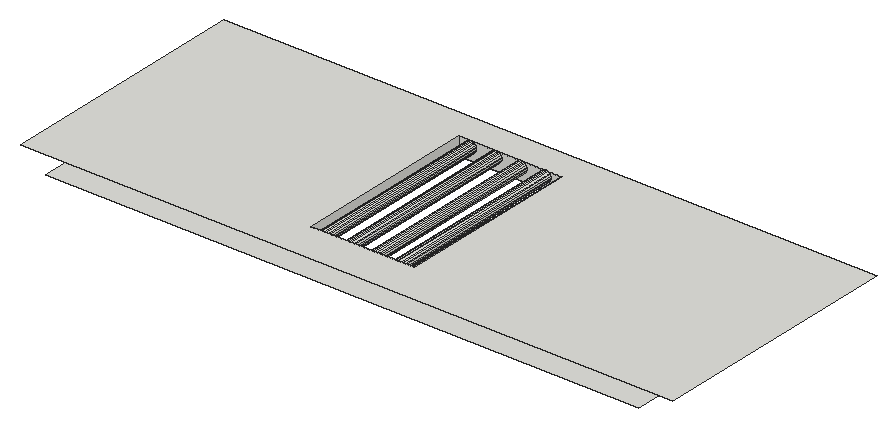
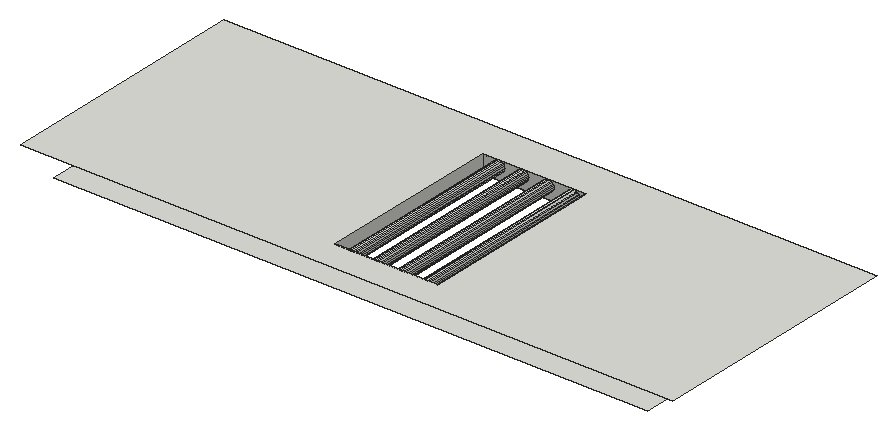
# SketchUp Ruby script. Lengths in inches.
U = 1.inch
M = Sketchup.active_model
def pt(a) = Geom::Point3d.new(a.map { |v| v * U })
def face(e, loops, mat)
  f = e.add_face(loops[0].map { |a| pt(a) })
  loops[1..].each { |l| e.add_face(l.map { |a| pt(a) }).erase! }
  f.material = f.back_material = mat if mat
  f
end
# faces: each face lists its corners as indices into pts; further lists are holes
def faces(e, pts, list, mat = nil) = list.each { |f| face(e, (f[0].is_a?(Array) ? f : [f]).map { |l| l.map { |i| pts[i] } }, mat) }
# xy, xz, yz: faces in a plane at the given z, y or x. An outline is a flat list of corners, or four numbers for a rectangle; further outlines are holes
def ring(l) = l.size == 4 ? [[l[0], l[1]], [l[2], l[1]], [l[2], l[3]], [l[0], l[3]]] : l.each_slice(2).to_a
def flat(e, list, mat, &to3) = list.each { |f| face(e, (f[0].is_a?(Array) ? f : [f]).map { |l| ring(l).map { |u, v| to3.(u, v) } }, mat) }
def xy(e, z, list, mat = nil) = flat(e, list, mat) { |x, y| [x, y, z] }
def xz(e, y, list, mat = nil) = flat(e, list, mat) { |x, z| [x, y, z] }
def yz(e, x, list, mat = nil) = flat(e, list, mat) { |y, z| [x, y, z] }
def lines(e, pts, list) = list.each { |a, b| e.add_line(pt(pts[a]), pt(pts[b])) }
# prism: a flat outline (further loops are holes) pulled along v
def prism(e, loops, v, mat = nil)
  f = face(e, loops, mat); d = Geom::Vector3d.new(v.map { |x| x * U })
  f.pushpull(f.normal.samedirection?(d) ? d.length : -d.length)
end
def box(e, o, s, mat = nil) = prism(e, [[o, [o[0] + s[0], o[1], o[2]], [o[0] + s[0], o[1] + s[1], o[2]], [o[0], o[1] + s[1], o[2]]]], [0, 0, s[2]], mat)
def at(x, y, z, deg = 0) = Geom::Transformation.translation(pt([x, y, z])) * Geom::Transformation.rotation(ORIGIN, Z_AXIS, deg.degrees)
def axes(o, x, y, z) = Geom::Transformation.new([*x, 0, *y, 0, *z, 0, *pt(o).to_a, 1])
def part(name) = M.definitions.add(name)
# library, detail: a bought-in or finely detailed component or shape, given as its bounding box
def library(name, o, s) = part(name).tap { |d| box(d.entities, o, s) }
def detail(e, o, s) = box(e.add_group.entities, o, s)
def put(e, d, t, mat = nil) = e.add_instance(d, t).tap { |i| i.material = mat if mat }
def group(e, t, mat = nil) = e.add_group.tap { |g| g.transformation = t; g.material = mat if mat }.entities
root = M.entities
xy(root,367.15,[[[9.02,53.875,221.54,144.86],[92.68,68.23,129.5,134.29],[86.02,110.58,86.54,110.6,87.04,110.74,87.48,111.01,87.84,111.39,88.09,111.85,88.22,112.36,88.2,112.88,88.06,113.38,87.79,113.83,87.41,114.1875,86.95,114.4375,86.44,114.56,85.92,114.55,85.42,114.4,84.97,114.13,84.61,113.75,84.36,113.29,84.24,112.78,84.25,112.26,84.4,111.76,84.67,111.32,85.05,110.96,85.51,110.71],[86.02,126.33,86.54,126.35,87.04,126.49,87.48,126.76,87.84,127.14,88.09,127.6,88.22,128.11,88.2,128.63,88.06,129.13,87.79,129.58,87.41,129.9375,86.95,130.1875,86.44,130.31,85.92,130.3,85.42,130.15,84.97,129.88,84.61,129.5,84.36,129.04,84.24,128.53,84.25,128.01,84.4,127.51,84.67,127.07,85.05,126.71,85.51,126.46],[86.02,95.96,86.54,95.97,87.04,96.12,87.48,96.39,87.84,96.77,88.09,97.23,88.22,97.73,88.2,98.26,88.06,98.76,87.79,99.2,87.41,99.5625,86.95,99.8125,86.44,99.94,85.92,99.92,85.42,99.78,84.97,99.5,84.61,99.125,84.36,98.67,84.24,98.16,84.25,97.64,84.4,97.14,84.67,96.69,85.05,96.33,85.51,96.08],[86.02,85.02,86.54,85.03,87.04,85.18,87.48,85.45,87.84,85.83,88.09,86.29,88.22,86.8,88.2,87.32,88.06,87.82,87.79,88.26,87.41,88.625,86.95,88.875,86.44,89,85.92,88.99,85.42,88.84,84.97,88.57,84.61,88.1875,84.36,87.73,84.24,87.22,84.25,86.7,84.4,86.2,84.67,85.75,85.05,85.39,85.51,85.14],[86.02,73.4,86.54,73.41,87.04,73.56,87.48,73.83,87.84,74.21,88.09,74.66,88.22,75.17,88.2,75.69,88.06,76.19,87.79,76.64,87.41,77,86.95,77.25,86.44,77.37,85.92,77.36,85.42,77.21,84.97,76.94,84.61,76.5625,84.36,76.1,84.24,75.6,84.25,75.08,84.4,74.57,84.67,74.13,85.05,73.77,85.51,73.52],[144.73,72.4,145.25,72.41,145.75,72.56,146.2,72.83,146.56,73.21,146.81,73.67,146.93,74.17,146.92,74.7,146.77,75.2,146.5,75.64,146.12,76,145.66,76.25,145.16,76.375,144.63,76.36,144.13,76.22,143.6875,75.94,143.33,75.57,143.08,75.11,142.95,74.6,142.97,74.08,143.11,73.58,143.39,73.13,143.76,72.77,144.22,72.52],[144.73,90.84,145.25,90.85,145.75,91,146.2,91.27,146.56,91.65,146.81,92.1,146.93,92.61,146.92,93.13,146.77,93.64,146.5,94.08,146.12,94.44,145.66,94.69,145.16,94.8125,144.63,94.8,144.13,94.65,143.6875,94.38,143.33,94,143.08,93.55,142.95,93.04,142.97,92.52,143.11,92.01,143.39,91.57,143.76,91.21,144.22,90.96],[144.73,112.15,145.25,112.16,145.75,112.31,146.2,112.58,146.56,112.96,146.81,113.42,146.93,113.92,146.92,114.45,146.77,114.95,146.5,115.39,146.12,115.75,145.66,116,145.16,116.125,144.63,116.11,144.13,115.97,143.6875,115.69,143.33,115.32,143.08,114.86,142.95,114.35,142.97,113.83,143.11,113.33,143.39,112.88,143.76,112.52,144.22,112.27],[144.73,130.65,145.25,130.66,145.75,130.81,146.2,131.08,146.56,131.46,146.81,131.92,146.93,132.42,146.92,132.95,146.77,133.45,146.5,133.89,146.12,134.25,145.66,134.5,145.16,134.625,144.63,134.61,144.13,134.47,143.6875,134.19,143.33,133.82,143.08,133.36,142.95,132.85,142.97,132.33,143.11,131.83,143.39,131.38,143.76,131.02,144.22,130.77]],[86.02,126.33,85.51,126.46,85.05,126.71,84.67,127.07,84.4,127.51,84.25,128.01,84.24,128.53,84.36,129.04,84.61,129.5,84.97,129.88,85.42,130.15,85.92,130.3,86.44,130.31,86.95,130.1875,87.41,129.9375,87.79,129.58,88.06,129.13,88.2,128.63,88.22,128.11,88.09,127.6,87.84,127.14,87.48,126.76,87.04,126.49,86.54,126.35]])
xy(root,367.77,[[144.73,112.15,144.22,112.27,143.76,112.52,143.39,112.88,143.11,113.33,142.97,113.83,142.95,114.35,143.08,114.86,143.33,115.32,143.6875,115.69,144.13,115.97,144.63,116.11,145.16,116.125,145.66,116,146.12,115.75,146.5,115.39,146.77,114.95,146.92,114.45,146.93,113.92,146.81,113.42,146.56,112.96,146.2,112.58,145.75,112.31,145.25,112.16],[144.73,130.65,144.22,130.77,143.76,131.02,143.39,131.38,143.11,131.83,142.97,132.33,142.95,132.85,143.08,133.36,143.33,133.82,143.6875,134.19,144.13,134.47,144.63,134.61,145.16,134.625,145.66,134.5,146.12,134.25,146.5,133.89,146.77,133.45,146.92,132.95,146.93,132.42,146.81,131.92,146.56,131.46,146.2,131.08,145.75,130.81,145.25,130.66]])
xy(root,368.02,[[86.02,85.02,85.51,85.14,85.05,85.39,84.67,85.75,84.4,86.2,84.25,86.7,84.24,87.22,84.36,87.73,84.61,88.1875,84.97,88.57,85.42,88.84,85.92,88.99,86.44,89,86.95,88.875,87.41,88.625,87.79,88.26,88.06,87.82,88.2,87.32,88.22,86.8,88.09,86.29,87.84,85.83,87.48,85.45,87.04,85.18,86.54,85.03]])
xy(root,368.27,[[86.02,95.96,85.51,96.08,85.05,96.33,84.67,96.69,84.4,97.14,84.25,97.64,84.24,98.16,84.36,98.67,84.61,99.125,84.97,99.5,85.42,99.78,85.92,99.92,86.44,99.94,86.95,99.8125,87.41,99.5625,87.79,99.2,88.06,98.76,88.2,98.26,88.22,97.73,88.09,97.23,87.84,96.77,87.48,96.39,87.04,96.12,86.54,95.97]])
xy(root,368.34,[[86.02,73.4,85.51,73.52,85.05,73.77,84.67,74.13,84.4,74.57,84.25,75.08,84.24,75.6,84.36,76.1,84.61,76.5625,84.97,76.94,85.42,77.21,85.92,77.36,86.44,77.37,86.95,77.25,87.41,77,87.79,76.64,88.06,76.19,88.2,75.69,88.22,75.17,88.09,74.66,87.84,74.21,87.48,73.83,87.04,73.56,86.54,73.41]])
xy(root,368.65,[[144.73,90.84,144.22,90.96,143.76,91.21,143.39,91.57,143.11,92.01,142.97,92.52,142.95,93.04,143.08,93.55,143.33,94,143.6875,94.38,144.13,94.65,144.63,94.8,145.16,94.8125,145.66,94.69,146.12,94.44,146.5,94.08,146.77,93.64,146.92,93.13,146.93,92.61,146.81,92.1,146.56,91.65,146.2,91.27,145.75,91,145.25,90.85]])
xy(root,369.46,[[86.02,110.58,85.51,110.71,85.05,110.96,84.67,111.32,84.4,111.76,84.25,112.26,84.24,112.78,84.36,113.29,84.61,113.75,84.97,114.13,85.42,114.4,85.92,114.55,86.44,114.56,86.95,114.4375,87.41,114.1875,87.79,113.83,88.06,113.38,88.2,112.88,88.22,112.36,88.09,111.85,87.84,111.39,87.48,111.01,87.04,110.74,86.54,110.6]])
xy(root,373.61,[[[0,53.875,233.71,144.86],[92.68,68.23,129.5,134.29]]])
xz(root,68.23,[[[92.68,367.15,129.5,373.61],[123.71,369.61,124.23,369.68,124.71,369.88,125.12,370.21,125.43,370.62,125.63,371.11,125.69,371.625,125.62,372.14,125.41,372.62,125.09,373.03,124.68,373.35,124.19,373.54,123.67,373.61,123.16,373.53,122.68,373.33,122.26,373.01,121.95,372.59,121.76,372.11,121.69,371.59,121.76,371.07,121.97,370.59,122.29,370.18,122.71,369.87,123.19,369.67]]])
xz(root,134.29,[[[92.68,367.15,129.5,373.61],[123.71,369.61,123.19,369.67,122.71,369.87,122.29,370.18,121.97,370.59,121.76,371.07,121.69,371.59,121.76,372.11,121.95,372.59,122.26,373.01,122.68,373.33,123.16,373.53,123.67,373.61,124.19,373.54,124.68,373.35,125.09,373.03,125.41,372.62,125.62,372.14,125.69,371.625,125.63,371.11,125.43,370.62,125.12,370.21,124.71,369.88,124.23,369.68]]])
yz(root,92.68,[[68.23,367.15,134.29,373.61]])
yz(root,129.5,[[68.23,367.15,134.29,373.61]])
p = [[86.02,73.4,367.15],[85.51,73.52,367.15],[85.51,73.52,368.34],[86.02,73.4,368.34],[86.54,73.41,367.15],[86.54,73.41,368.34],
  [87.04,73.56,367.15],[87.04,73.56,368.34],[85.05,73.77,367.15],[85.05,73.77,368.34],[87.48,73.83,367.15],[87.48,73.83,368.34],
  [84.67,74.13,367.15],[84.67,74.13,368.34],[87.84,74.21,367.15],[87.84,74.21,368.34],[84.4,74.57,367.15],[84.4,74.57,368.34],
  [88.09,74.66,367.15],[88.09,74.66,368.34],[84.25,75.08,367.15],[84.25,75.08,368.34],[88.22,75.17,367.15],[88.22,75.17,368.34],
  [84.24,75.6,367.15],[84.24,75.6,368.34],[88.2,75.69,367.15],[88.2,75.69,368.34],[84.36,76.1,367.15],[84.36,76.1,368.34],
  [88.06,76.19,367.15],[88.06,76.19,368.34],[84.61,76.5625,367.15],[84.61,76.5625,368.34],[87.79,76.64,367.15],[87.79,76.64,368.34],
  [84.97,76.94,367.15],[84.97,76.94,368.34],[87.41,77,367.15],[87.41,77,368.34],[85.42,77.21,367.15],[85.42,77.21,368.34],
  [86.95,77.25,367.15],[86.95,77.25,368.34],[85.92,77.36,367.15],[85.92,77.36,368.34],[86.44,77.37,367.15],[86.44,77.37,368.34],
  [86.02,85.02,367.15],[85.51,85.14,367.15],[85.51,85.14,368.02],[86.02,85.02,368.02],[86.54,85.03,367.15],[86.54,85.03,368.02],
  [87.04,85.18,367.15],[87.04,85.18,368.02],[85.05,85.39,367.15],[85.05,85.39,368.02],[87.48,85.45,367.15],[87.48,85.45,368.02],
  [84.67,85.75,367.15],[84.67,85.75,368.02],[87.84,85.83,367.15],[87.84,85.83,368.02],[84.4,86.2,367.15],[84.4,86.2,368.02],
  [88.09,86.29,367.15],[88.09,86.29,368.02],[84.25,86.7,367.15],[84.25,86.7,368.02],[88.22,86.8,367.15],[88.22,86.8,368.02],
  [84.24,87.22,367.15],[84.24,87.22,368.02],[88.2,87.32,367.15],[88.2,87.32,368.02],[84.36,87.73,367.15],[84.36,87.73,368.02],
  [88.06,87.82,367.15],[88.06,87.82,368.02],[84.61,88.1875,367.15],[84.61,88.1875,368.02],[87.79,88.26,367.15],[87.79,88.26,368.02],
  [84.97,88.57,367.15],[84.97,88.57,368.02],[87.41,88.625,367.15],[87.41,88.625,368.02],[85.42,88.84,367.15],[85.42,88.84,368.02],
  [86.95,88.875,367.15],[86.95,88.875,368.02],[85.92,88.99,367.15],[85.92,88.99,368.02],[86.44,89,367.15],[86.44,89,368.02],
  [144.73,90.84,368.65],[144.73,90.84,367.15],[144.22,90.96,367.15],[144.22,90.96,368.65],[145.25,90.85,368.65],[145.25,90.85,367.15],
  [145.75,91,368.65],[145.75,91,367.15],[143.76,91.21,367.15],[143.76,91.21,368.65],[146.2,91.27,368.65],[146.2,91.27,367.15],
  [143.39,91.57,367.15],[143.39,91.57,368.65],[146.56,91.65,368.65],[146.56,91.65,367.15],[143.11,92.01,367.15],[143.11,92.01,368.65],
  [146.81,92.1,368.65],[146.81,92.1,367.15],[142.97,92.52,367.15],[142.97,92.52,368.65],[146.93,92.61,368.65],[146.93,92.61,367.15],
  [142.95,93.04,367.15],[142.95,93.04,368.65],[146.92,93.13,368.65],[146.92,93.13,367.15],[143.08,93.55,367.15],[143.08,93.55,368.65],
  [146.77,93.64,368.65],[146.77,93.64,367.15],[143.33,94,367.15],[143.33,94,368.65],[146.5,94.08,368.65],[146.5,94.08,367.15],
  [143.6875,94.38,367.15],[143.6875,94.38,368.65],[146.12,94.44,368.65],[146.12,94.44,367.15],[144.13,94.65,367.15],[144.13,94.65,368.65],
  [145.66,94.69,368.65],[145.66,94.69,367.15],[144.63,94.8,367.15],[144.63,94.8,368.65],[145.16,94.8125,368.65],[145.16,94.8125,367.15],
  [86.02,95.96,367.15],[85.51,96.08,367.15],[85.51,96.08,368.27],[86.02,95.96,368.27],[86.54,95.97,367.15],[86.54,95.97,368.27],
  [87.04,96.12,367.15],[87.04,96.12,368.27],[85.05,96.33,367.15],[85.05,96.33,368.27],[87.48,96.39,367.15],[87.48,96.39,368.27],
  [84.67,96.69,367.15],[84.67,96.69,368.27],[87.84,96.77,367.15],[87.84,96.77,368.27],[84.4,97.14,367.15],[84.4,97.14,368.27],
  [88.09,97.23,367.15],[88.09,97.23,368.27],[84.25,97.64,367.15],[84.25,97.64,368.27],[88.22,97.73,367.15],[88.22,97.73,368.27],
  [84.24,98.16,367.15],[84.24,98.16,368.27],[88.2,98.26,367.15],[88.2,98.26,368.27],[84.36,98.67,367.15],[84.36,98.67,368.27],
  [88.06,98.76,367.15],[88.06,98.76,368.27],[84.61,99.125,367.15],[84.61,99.125,368.27],[87.79,99.2,367.15],[87.79,99.2,368.27],
  [84.97,99.5,367.15],[84.97,99.5,368.27],[87.41,99.5625,367.15],[87.41,99.5625,368.27],[85.42,99.78,367.15],[85.42,99.78,368.27],
  [86.95,99.8125,367.15],[86.95,99.8125,368.27],[85.92,99.92,367.15],[85.92,99.92,368.27],[86.44,99.94,367.15],[86.44,99.94,368.27],
  [86.02,110.58,367.15],[85.51,110.71,367.15],[85.51,110.71,369.46],[86.02,110.58,369.46],[86.54,110.6,367.15],[86.54,110.6,369.46],
  [87.04,110.74,367.15],[87.04,110.74,369.46],[85.05,110.96,367.15],[85.05,110.96,369.46],[87.48,111.01,367.15],[87.48,111.01,369.46],
  [84.67,111.32,367.15],[84.67,111.32,369.46],[87.84,111.39,367.15],[87.84,111.39,369.46],[84.4,111.76,367.15],[84.4,111.76,369.46],
  [88.09,111.85,367.15],[88.09,111.85,369.46],[84.25,112.26,367.15],[84.25,112.26,369.46],[88.22,112.36,367.15],[88.22,112.36,369.46],
  [144.22,112.27,367.77],[144.73,112.15,367.77],[144.73,112.15,367.15],[144.22,112.27,367.15],[145.25,112.16,367.77],[145.25,112.16,367.15],
  [145.75,112.31,367.77],[145.75,112.31,367.15],[84.24,112.78,367.15],[84.24,112.78,369.46],[143.76,112.52,367.77],[143.76,112.52,367.15],
  [146.2,112.58,367.77],[146.2,112.58,367.15],[88.2,112.88,367.15],[88.2,112.88,369.46],[143.39,112.88,367.77],[143.39,112.88,367.15],
  [146.56,112.96,367.77],[146.56,112.96,367.15],[84.36,113.29,367.15],[84.36,113.29,369.46],[88.06,113.38,367.15],[88.06,113.38,369.46],
  [143.11,113.33,367.77],[143.11,113.33,367.15],[146.81,113.42,367.77],[146.81,113.42,367.15],[84.61,113.75,367.15],[84.61,113.75,369.46],
  [142.97,113.83,367.77],[142.97,113.83,367.15],[87.79,113.83,367.15],[87.79,113.83,369.46],[146.93,113.92,367.77],[146.93,113.92,367.15],
  [84.97,114.13,367.15],[84.97,114.13,369.46],[87.41,114.1875,367.15],[87.41,114.1875,369.46],[142.95,114.35,367.77],[142.95,114.35,367.15],
  [146.92,114.45,367.77],[146.92,114.45,367.15],[85.42,114.4,367.15],[85.42,114.4,369.46],[86.95,114.4375,367.15],[86.95,114.4375,369.46],
  [85.92,114.55,367.15],[85.92,114.55,369.46],[86.44,114.56,367.15],[86.44,114.56,369.46],[143.08,114.86,367.77],[143.08,114.86,367.15],
  [146.77,114.95,367.77],[146.77,114.95,367.15],[143.33,115.32,367.77],[143.33,115.32,367.15],[146.5,115.39,367.77],[146.5,115.39,367.15],
  [143.6875,115.69,367.77],[143.6875,115.69,367.15],[146.12,115.75,367.77],[146.12,115.75,367.15],[144.13,115.97,367.77],[144.13,115.97,367.15],
  [145.66,116,367.77],[145.66,116,367.15],[144.63,116.11,367.77],[144.63,116.11,367.15],[145.16,116.125,367.77],[145.16,116.125,367.15],
  [144.22,130.77,367.77],[144.73,130.65,367.77],[144.73,130.65,367.15],[144.22,130.77,367.15],[145.25,130.66,367.77],[145.25,130.66,367.15],
  [145.75,130.81,367.77],[145.75,130.81,367.15],[143.76,131.02,367.77],[143.76,131.02,367.15],[146.2,131.08,367.77],[146.2,131.08,367.15],
  [143.39,131.38,367.77],[143.39,131.38,367.15],[146.56,131.46,367.77],[146.56,131.46,367.15],[143.11,131.83,367.77],[143.11,131.83,367.15],
  [146.81,131.92,367.77],[146.81,131.92,367.15],[142.97,132.33,367.77],[142.97,132.33,367.15],[146.93,132.42,367.77],[146.93,132.42,367.15],
  [142.95,132.85,367.77],[142.95,132.85,367.15],[146.92,132.95,367.77],[146.92,132.95,367.15],[143.08,133.36,367.77],[143.08,133.36,367.15],
  [146.77,133.45,367.77],[146.77,133.45,367.15],[143.33,133.82,367.77],[143.33,133.82,367.15],[146.5,133.89,367.77],[146.5,133.89,367.15],
  [143.6875,134.19,367.77],[143.6875,134.19,367.15],[146.12,134.25,367.77],[146.12,134.25,367.15],[144.13,134.47,367.77],[144.13,134.47,367.15],
  [145.66,134.5,367.77],[145.66,134.5,367.15],[144.63,134.61,367.77],[144.63,134.61,367.15],[145.16,134.625,367.77],[145.16,134.625,367.15],
  [96.44,134.29,369.67],[96.96,134.29,369.61],[96.96,68.23,369.61],[96.44,68.23,369.67],[97.48,134.29,369.68],[97.48,68.23,369.68],
  [105.5,134.29,369.67],[106.02,134.29,369.61],[106.02,68.23,369.61],[105.5,68.23,369.67],[106.54,134.29,369.68],[106.54,68.23,369.68],
  [114.57,134.29,369.67],[115.08,134.29,369.61],[115.08,68.23,369.61],[114.57,68.23,369.67],[115.6,134.29,369.68],[115.6,68.23,369.68],
  [123.19,134.29,369.67],[123.71,134.29,369.61],[123.71,68.23,369.61],[123.19,68.23,369.67],[124.23,134.29,369.68],[124.23,68.23,369.68],
  [95.96,134.29,369.87],[95.96,68.23,369.87],[97.96,134.29,369.88],[97.96,68.23,369.88],[105.02,134.29,369.87],[105.02,68.23,369.87],
  [107.02,134.29,369.88],[107.02,68.23,369.88],[114.08,134.29,369.87],[114.08,68.23,369.87],[116.08,134.29,369.88],[116.08,68.23,369.88],
  [122.71,134.29,369.87],[122.71,68.23,369.87],[124.71,134.29,369.88],[124.71,68.23,369.88],[95.54,134.29,370.18],[95.54,68.23,370.18],
  [98.37,134.29,370.21],[98.37,68.23,370.21],[104.6,134.29,370.18],[104.6,68.23,370.18],[107.43,134.29,370.21],[107.43,68.23,370.21],
  [113.67,134.29,370.18],[113.67,68.23,370.18],[116.49,134.29,370.21],[116.49,68.23,370.21],[122.29,134.29,370.18],[122.29,68.23,370.18],
  [125.12,134.29,370.21],[125.12,68.23,370.21],[95.22,134.29,370.59],[95.22,68.23,370.59],[98.68,134.29,370.62],[98.68,68.23,370.62],
  [104.28,134.29,370.59],[104.28,68.23,370.59],[107.75,134.29,370.62],[107.75,68.23,370.62],[113.34,134.29,370.59],[113.34,68.23,370.59],
  [116.81,134.29,370.62],[116.81,68.23,370.62],[121.97,134.29,370.59],[121.97,68.23,370.59],[125.43,134.29,370.62],[125.43,68.23,370.62],
  [95.01,134.29,371.07],[95.01,68.23,371.07],[98.88,134.29,371.11],[98.88,68.23,371.11],[104.08,134.29,371.07],[104.08,68.23,371.07],
  [107.94,134.29,371.11],[107.94,68.23,371.11],[113.14,134.29,371.07],[113.14,68.23,371.07],[117,134.29,371.11],[117,68.23,371.11],
  [121.76,134.29,371.07],[121.76,68.23,371.07],[125.63,134.29,371.11],[125.63,68.23,371.11],[94.94,134.29,371.59],[94.94,68.23,371.59],
  [98.94,134.29,371.625],[98.94,68.23,371.625],[104,134.29,371.59],[104,68.23,371.59],[108,134.29,371.625],[108,68.23,371.625],
  [113.07,134.29,371.59],[113.07,68.23,371.59],[117.07,134.29,371.625],[117.07,68.23,371.625],[121.69,134.29,371.59],[121.69,68.23,371.59],
  [125.69,134.29,371.625],[125.69,68.23,371.625],[95.01,134.29,372.11],[95.01,68.23,372.11],[98.87,134.29,372.14],[98.87,68.23,372.14],
  [104.07,134.29,372.11],[104.07,68.23,372.11],[107.93,134.29,372.14],[107.93,68.23,372.14],[113.13,134.29,372.11],[113.13,68.23,372.11],
  [116.99,134.29,372.14],[116.99,68.23,372.14],[121.76,134.29,372.11],[121.76,68.23,372.11],[125.62,134.29,372.14],[125.62,68.23,372.14],
  [95.2,134.29,372.59],[95.2,68.23,372.59],[98.66,134.29,372.62],[98.66,68.23,372.62],[104.26,134.29,372.59],[104.26,68.23,372.59],
  [107.73,134.29,372.62],[107.73,68.23,372.62],[113.33,134.29,372.59],[113.33,68.23,372.59],[116.79,134.29,372.62],[116.79,68.23,372.62],
  [121.95,134.29,372.59],[121.95,68.23,372.59],[125.41,134.29,372.62],[125.41,68.23,372.62],[95.51,134.29,373.01],[95.51,68.23,373.01],
  [98.34,134.29,373.03],[98.34,68.23,373.03],[104.58,134.29,373.01],[104.58,68.23,373.01],[107.41,134.29,373.03],[107.41,68.23,373.03],
  [113.64,134.29,373.01],[113.64,68.23,373.01],[116.47,134.29,373.03],[116.47,68.23,373.03],[122.26,134.29,373.01],[122.26,68.23,373.01],
  [125.09,134.29,373.03],[125.09,68.23,373.03],[95.93,134.29,373.33],[95.93,68.23,373.33],[97.93,134.29,373.35],[97.93,68.23,373.35],
  [104.99,134.29,373.33],[104.99,68.23,373.33],[106.99,134.29,373.35],[106.99,68.23,373.35],[114.05,134.29,373.33],[114.05,68.23,373.33],
  [116.05,134.29,373.35],[116.05,68.23,373.35],[122.68,134.29,373.33],[122.68,68.23,373.33],[124.68,134.29,373.35],[124.68,68.23,373.35],
  [96.41,134.29,373.53],[96.41,68.23,373.53],[97.44,134.29,373.54],[97.44,68.23,373.54],[105.47,134.29,373.53],[105.47,68.23,373.53],
  [106.5,134.29,373.54],[106.5,68.23,373.54],[114.53,134.29,373.53],[114.53,68.23,373.53],[115.57,134.29,373.54],[115.57,68.23,373.54],
  [123.16,134.29,373.53],[123.16,68.23,373.53],[124.19,134.29,373.54],[124.19,68.23,373.54],[96.92,134.29,373.61],[96.92,68.23,373.61],
  [105.99,134.29,373.61],[105.99,68.23,373.61],[115.05,134.29,373.61],[115.05,68.23,373.61],[123.67,134.29,373.61],[123.67,68.23,373.61]]
faces(root,p,[[0,1,2,3],[4,0,3,5],[6,4,5,7],[1,8,9,2],[10,6,7,11],[8,12,13,9],[14,10,11,15],[12,16,17,13],
  [18,14,15,19],[16,20,21,17],[22,18,19,23],[20,24,25,21],[26,22,23,27],[24,28,29,25],[30,26,27,31],[28,32,33,29],
  [34,30,31,35],[32,36,37,33],[38,34,35,39],[36,40,41,37],[42,38,39,43],[40,44,45,41],[46,42,43,47],[44,46,47,45],
  [48,49,50,51],[52,48,51,53],[54,52,53,55],[49,56,57,50],[58,54,55,59],[56,60,61,57],[62,58,59,63],[60,64,65,61],
  [66,62,63,67],[64,68,69,65],[70,66,67,71],[68,72,73,69],[74,70,71,75],[72,76,77,73],[78,74,75,79],[76,80,81,77],
  [82,78,79,83],[80,84,85,81],[86,82,83,87],[84,88,89,85],[90,86,87,91],[88,92,93,89],[94,90,91,95],[92,94,95,93],
  [96,97,98,99],[100,101,97,96],[102,103,101,100],[99,98,104,105],[106,107,103,102],[105,104,108,109],[110,111,107,106],[109,108,112,113],
  [114,115,111,110],[113,112,116,117],[118,119,115,114],[117,116,120,121],[122,123,119,118],[121,120,124,125],[126,127,123,122],[125,124,128,129],
  [130,131,127,126],[129,128,132,133],[134,135,131,130],[133,132,136,137],[138,139,135,134],[137,136,140,141],[142,143,139,138],[141,140,143,142],
  [144,145,146,147],[148,144,147,149],[150,148,149,151],[145,152,153,146],[154,150,151,155],[152,156,157,153],[158,154,155,159],[156,160,161,157],
  [162,158,159,163],[160,164,165,161],[166,162,163,167],[164,168,169,165],[170,166,167,171],[168,172,173,169],[174,170,171,175],[172,176,177,173],
  [178,174,175,179],[176,180,181,177],[182,178,179,183],[180,184,185,181],[186,182,183,187],[184,188,189,185],[190,186,187,191],[188,190,191,189],
  [192,193,194,195],[196,192,195,197],[198,196,197,199],[193,200,201,194],[202,198,199,203],[200,204,205,201],[206,202,203,207],[204,208,209,205],
  [210,206,207,211],[208,212,213,209],[214,210,211,215],[216,217,218,219],[217,220,221,218],[220,222,223,221],[212,224,225,213],[226,216,219,227],
  [222,228,229,223],[230,214,215,231],[232,226,227,233],[228,234,235,229],[224,236,237,225],[238,230,231,239],[240,232,233,241],[234,242,243,235],
  [236,244,245,237],[246,240,241,247],[248,238,239,249],[242,250,251,243],[244,252,253,245],[254,248,249,255],[256,246,247,257],[250,258,259,251],
  [252,260,261,253],[262,254,255,263],[260,264,265,261],[266,262,263,267],[268,256,257,269],[258,270,271,259],[264,266,267,265],[272,268,269,273],
  [270,274,275,271],[276,272,273,277],[274,278,279,275],[280,276,277,281],[278,282,283,279],[284,280,281,285],[282,286,287,283],[286,284,285,287],
  [288,289,290,291],[289,292,293,290],[292,294,295,293],[296,288,291,297],[294,298,299,295],[300,296,297,301],[298,302,303,299],[304,300,301,305],
  [302,306,307,303],[308,304,305,309],[306,310,311,307],[312,308,309,313],[310,314,315,311],[316,312,313,317],[314,318,319,315],[320,316,317,321],
  [318,322,323,319],[324,320,321,325],[322,326,327,323],[328,324,325,329],[326,330,331,327],[332,328,329,333],[330,334,335,331],[334,332,333,335],
  [336,337,338,339],[337,340,341,338],[342,343,344,345],[343,346,347,344],[348,349,350,351],[349,352,353,350],[354,355,356,357],[355,358,359,356],
  [360,336,339,361],[340,362,363,341],[364,342,345,365],[346,366,367,347],[368,348,351,369],[352,370,371,353],[372,354,357,373],[358,374,375,359],
  [376,360,361,377],[362,378,379,363],[380,364,365,381],[366,382,383,367],[384,368,369,385],[370,386,387,371],[388,372,373,389],[374,390,391,375],
  [392,376,377,393],[378,394,395,379],[396,380,381,397],[382,398,399,383],[400,384,385,401],[386,402,403,387],[404,388,389,405],[390,406,407,391],
  [408,392,393,409],[394,410,411,395],[412,396,397,413],[398,414,415,399],[416,400,401,417],[402,418,419,403],[420,404,405,421],[406,422,423,407],
  [424,408,409,425],[410,426,427,411],[428,412,413,429],[414,430,431,415],[432,416,417,433],[418,434,435,419],[436,420,421,437],[422,438,439,423],
  [440,424,425,441],[426,442,443,427],[444,428,429,445],[430,446,447,431],[448,432,433,449],[434,450,451,435],[452,436,437,453],[438,454,455,439],
  [456,440,441,457],[442,458,459,443],[460,444,445,461],[446,462,463,447],[464,448,449,465],[450,466,467,451],[468,452,453,469],[454,470,471,455],
  [472,456,457,473],[458,474,475,459],[476,460,461,477],[462,478,479,463],[480,464,465,481],[466,482,483,467],[484,468,469,485],[470,486,487,471],
  [488,472,473,489],[474,490,491,475],[492,476,477,493],[478,494,495,479],[496,480,481,497],[482,498,499,483],[500,484,485,501],[486,502,503,487],
  [504,488,489,505],[490,506,507,491],[508,492,493,509],[494,510,511,495],[512,496,497,513],[498,514,515,499],[516,500,501,517],[502,518,519,503],
  [520,504,505,521],[506,520,521,507],[522,508,509,523],[510,522,523,511],[524,512,513,525],[514,524,525,515],[526,516,517,527],[518,526,527,519]])
